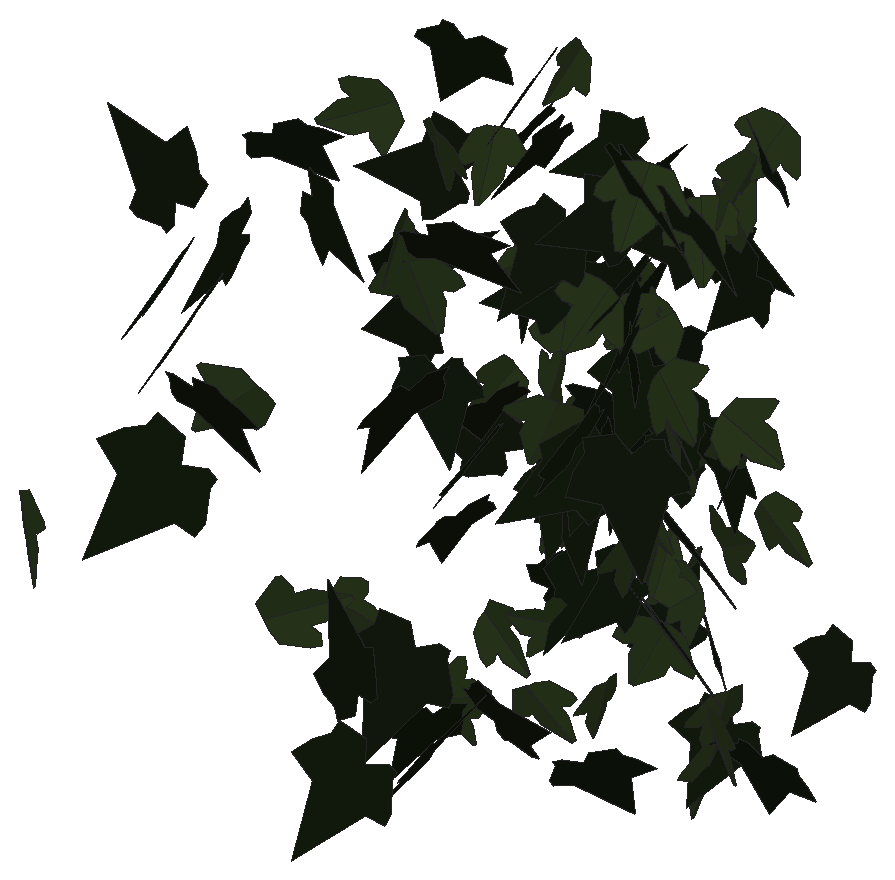
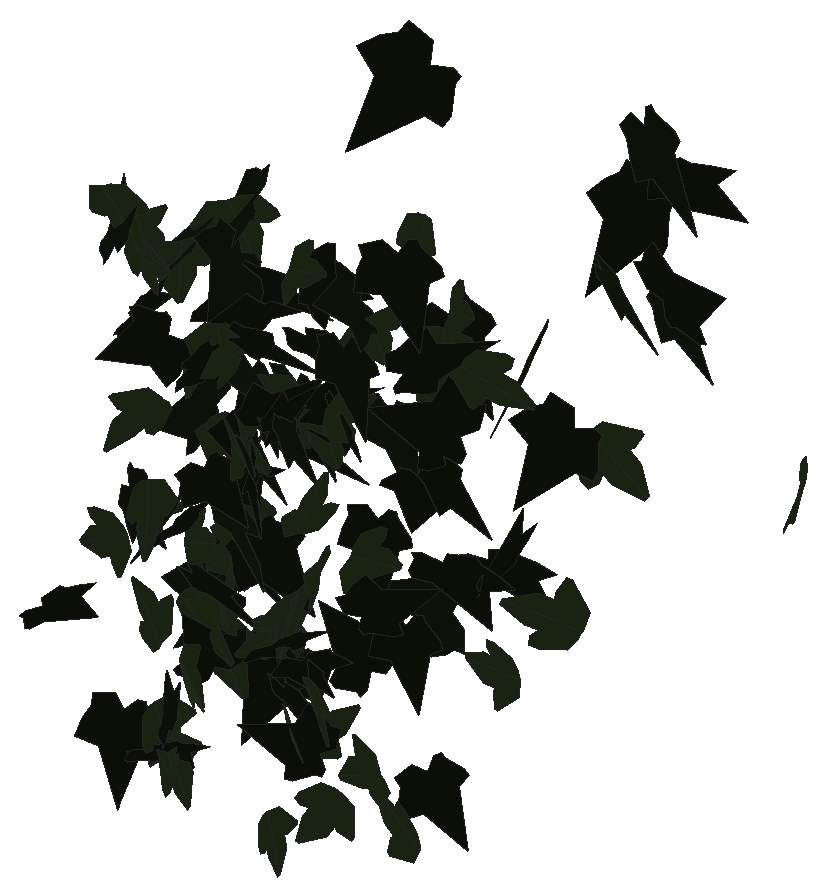
# SketchUp Ruby script. Lengths in inches.
U = 1.inch
M = Sketchup.active_model
def pt(a) = Geom::Point3d.new(a.map { |v| v * U })
def face(e, loops, mat)
  f = e.add_face(loops[0].map { |a| pt(a) })
  loops[1..].each { |l| e.add_face(l.map { |a| pt(a) }).erase! }
  f.material = f.back_material = mat if mat
  f
end
# faces: each face lists its corners as indices into pts; further lists are holes
def faces(e, pts, list, mat = nil) = list.each { |f| face(e, (f[0].is_a?(Array) ? f : [f]).map { |l| l.map { |i| pts[i] } }, mat) }
# xy, xz, yz: faces in a plane at the given z, y or x. An outline is a flat list of corners, or four numbers for a rectangle; further outlines are holes
def ring(l) = l.size == 4 ? [[l[0], l[1]], [l[2], l[1]], [l[2], l[3]], [l[0], l[3]]] : l.each_slice(2).to_a
def flat(e, list, mat, &to3) = list.each { |f| face(e, (f[0].is_a?(Array) ? f : [f]).map { |l| ring(l).map { |u, v| to3.(u, v) } }, mat) }
def xy(e, z, list, mat = nil) = flat(e, list, mat) { |x, y| [x, y, z] }
def xz(e, y, list, mat = nil) = flat(e, list, mat) { |x, z| [x, y, z] }
def yz(e, x, list, mat = nil) = flat(e, list, mat) { |y, z| [x, y, z] }
def lines(e, pts, list) = list.each { |a, b| e.add_line(pt(pts[a]), pt(pts[b])) }
# prism: a flat outline (further loops are holes) pulled along v
def prism(e, loops, v, mat = nil)
  f = face(e, loops, mat); d = Geom::Vector3d.new(v.map { |x| x * U })
  f.pushpull(f.normal.samedirection?(d) ? d.length : -d.length)
end
def box(e, o, s, mat = nil) = prism(e, [[o, [o[0] + s[0], o[1], o[2]], [o[0] + s[0], o[1] + s[1], o[2]], [o[0], o[1] + s[1], o[2]]]], [0, 0, s[2]], mat)
def at(x, y, z, deg = 0) = Geom::Transformation.translation(pt([x, y, z])) * Geom::Transformation.rotation(ORIGIN, Z_AXIS, deg.degrees)
def axes(o, x, y, z) = Geom::Transformation.new([*x, 0, *y, 0, *z, 0, *pt(o).to_a, 1])
def part(name) = M.definitions.add(name)
# library, detail: a bought-in or finely detailed component or shape, given as its bounding box
def library(name, o, s) = part(name).tap { |d| box(d.entities, o, s) }
def detail(e, o, s) = box(e.add_group.entities, o, s)
def put(e, d, t, mat = nil) = e.add_instance(d, t).tap { |i| i.material = mat if mat }
def group(e, t, mat = nil) = e.add_group.tap { |g| g.transformation = t; g.material = mat if mat }.entities
root = M.entities
M.materials.add("efeu1").color = [18, 25, 13]
M.materials.add("efeu2").color = [43, 57, 29]
c1 = part("ivyleaf_9")
p = [[1.54,2.16,1.25],[1.36,2.04,1.19],[-0.21,0.99,0.68],[-0.71,1.11,0.82],[-0.85,0.86,0.67],[-0.8,0.17,0.21],
  [-0.9,-0.01,0.1],[-0.67,-0.16,-0.02],[-0.08,-0.08,-0.05],[-0.03,-0.6,-0.4],[0.65,-0.88,-0.66],[0.83,-0.6,-0.49],
  [1.29,-0.42,-0.43],[1.8125,-0.07,-0.26],[1.21,0.44,0.15]]
faces(c1.entities,p,[[0,1,2,3,4,5,6,7,8,9,10,11,12,13,14]],"efeu1")
c2 = part("ivyleaf_10")
p = [[0,0.5,-0.03],[-0.0625,2.02,-0.43],[-0.19,2.01,-0.46],[-0.54,1.05,-0.29],[-0.52,0.625,-0.18],[-0.83,0.76,-0.28],
  [-1.16,0.64,-0.33],[-1.15,0.33,-0.24],[-0.77,-0.39,0.02],[-0.3,-0.51,0.16],[0.04,-0.48,0.23],[-0.02,2.01,-0.4375],
  [-0.06,2.01,-0.43],[0.04,-0.49,0.23],[0.67,-0.49,0.14],[1.38,0.36,-0.2],[1.375,0.51,-0.24],[0.81,0.65,-0.19],
  [0.62,0.59,-0.15],[0.6,1.09,-0.28],[0.5,1.23,-0.31]]
faces(c2.entities,p,[[0,1,2,3,4,5,6,7,8,9,10],[11,12,0,13,14,15,16,17,18,19,20]],"efeu2")
put(root,c1,axes([502.58,109.68,200.72],[-1.12448,-0.74552,0.3301],[-0.2858,-0.17561,-1.33175],[0.82712,-1.07423,-0.01139]))
put(root,c1,axes([501.1,112.36,204.29],[-0.7784,0.97057,-0.39309],[0.24336,-0.30345,-1.25727],[-1.09825,-0.75515,0.00001]))
put(root,c1,axes([501.125,112.48,201.625],[1.28442,0.17447,-0.3013],[-0.30972,-0.0411,-1.25008],[-0.19359,1.22336,0.00097]))
put(root,c2,axes([493.45,113.83,194.24],[-0.39891,0.91131,-0.49784],[0.20278,-0.4404,-1.02262],[-1.09308,-0.41427,-0.00803]))
put(root,c1,axes([504.72,115.95,188.35],[-1.14523,-0.49988,-0.02559],[0.0231,0.01234,-1.2192],[0.54003,-1.06061,-0.00212]))
put(root,c1,axes([496.22,117.38,201.86],[-0.6941,0.75659,-0.35945],[0.22061,-0.27983,-1.03212],[-0.87083,-0.67394,0.02503]))
put(root,c1,axes([506.59,117.12,206.83],[1.24321,0.52526,0.11586],[0.07008,0.12552,-1.3128],[-0.57565,1.14967,0.09039]))
put(root,c1,axes([502.87,117.99,189.51],[-0.31457,-0.86412,0.68269],[0.21886,0.6244,0.94834],[-1.15137,0.35478,-0.00626]))
put(root,c1,axes([497.61,118.89,202.94],[-0.9682,0.4916,-0.3634],[0.31268,-0.19839,-1.06277],[-0.57143,-0.9415,0.03419]))
put(root,c1,axes([504.9,118.04,187.32],[-0.23729,1.03065,-0.31438],[-0.06927,0.29541,1.09596],[1.15792,0.22888,0.00114]))
put(root,c1,axes([503.63,119.76,190.27],[-1.1445,-0.59034,-0.29556],[0.2678,0.13885,-1.26158],[0.65497,-1.08834,-0.00063]))
put(root,c1,axes([503.72,119.43,199.4],[-0.28753,0.99191,-0.63209],[0.14608,-0.59287,-1.0679],[-1.24785,-0.29796,0.02063]))
put(root,c2,axes([497.17,119.74,197],[-0.65814,-0.39458,0.80063],[-0.66489,-0.46373,-0.75402],[0.65635,-0.86542,0.03899]))
put(root,c1,axes([494.78,119.24,203.17],[-0.07387,0.16981,1.26175],[-0.9393,0.84901,-0.17458],[-0.93176,-0.86935,0.07597]))
put(root,c2,axes([498.64,119.69,189.78],[-0.30008,-0.31215,0.99531],[0.67558,0.72433,0.43458],[-0.8518,0.68444,-0.00597]))
put(root,c1,axes([510.7,121.53,198.65],[-0.42664,-1.05008,-0.53356],[0.14703,0.49652,-1.16594],[1.25361,-0.41561,-0.04484]))
put(root,c1,axes([504.47,121.55,196.39],[-0.46469,1.05397,0.07174],[-0.02966,0.06329,-1.18395],[-1.14033,-0.43114,0.00156]))
put(root,c1,axes([504.78,122.39,187.17],[0.11824,-0.4021,0.99356],[0.82864,-0.61447,-0.36042],[0.75267,0.73966,0.24072]))
put(root,c2,axes([498.83,122.57,189.05],[-0.10427,0.04499,-0.96535],[0.9176,-0.3738,-0.11075],[-0.40661,-0.8551,-0.00238]))
put(root,c2,axes([500.64,123.125,202.36],[-0.12804,0.53057,-0.80239],[-0.0198,-0.77885,-0.5541],[-1.01107,-0.05194,0.11246]))
put(root,c1,axes([508.03,122.69,186.64],[0.8456,0.75683,-0.05717],[-0.04278,-0.03812,-1.13251],[-0.81841,0.78396,0.00013]))
put(root,c2,axes([500.99,123.17,200.95],[-1.0217,-0.4777,-0.27537],[0.26785,0.0961,-1.10186],[0.52554,-0.97766,0.02624]))
put(root,c1,axes([507.25,123.02,197.17],[-0.57036,1.00267,0.20462],[-0.15002,0.14897,-1.1773],[-1.09329,-0.54352,0.05479]))
put(root,c1,axes([497.16,123.13,202.18],[0.78046,-0.5228,-0.7206],[-0.58139,0.4373,-0.92706],[0.73537,0.90059,0.03185]))
put(root,c1,axes([510.3125,123.64,195.68],[0.93816,-0.72233,0.31366],[0.26081,-0.18126,-1.17485],[0.80415,0.90149,0.0151]))
put(root,c1,axes([506.99,124.13,196.03],[-1.19107,-0.1307,0.24865],[-0.24665,-0.10024,-1.15262],[0.1605,-1.124,0.07388]))
put(root,c1,axes([500.93,124.04,185.1875],[-0.10999,0.70293,-0.64495],[0.05457,-0.61877,-0.73806],[-1.0109,-0.10988,0.03033]))
put(root,c2,axes([505.6,124.12,197.34],[-0.72728,-0.6263,0.36516],[-0.26936,-0.24736,-0.95636],[0.72716,-0.71803,0.01096]))
put(root,c2,axes([501.51,123.8,205.4375],[-0.89854,0.37381,0.22973],[-0.2145,0.09692,-0.94856],[-0.417,-0.85533,-0.00709]))
put(root,c1,axes([507.2,125.03,196.22],[0.24883,-0.17622,-1.1552],[1.0631,-0.51682,0.29761],[-0.5875,-1.00984,0.04927]))
put(root,c1,axes([500.62,124.75,196.65],[-0.52574,-0.57982,-0.59905],[0.4189,0.42623,-0.78712],[0.77694,-0.62216,0.01903]))
put(root,c1,axes([508.86,125.45,190.45],[0.69979,-0.69154,0.50361],[0.36067,-0.35067,-0.98556],[0.83739,0.72894,0.00364]))
put(root,c2,axes([507.82,125.28,193.22],[0.00137,-1.07638,-0.0221],[0.02048,0.02126,-1.11926],[1.16254,0.00089,0.01975]))
put(root,c1,axes([507.43,125.55,191.58],[-1.10582,0.27068,-0.05513],[0.05405,-0.01809,-1.10144],[-0.29294,-1.02512,0.00488]))
put(root,c2,axes([509.33,124.99,199.16],[0.05607,0.98769,0.41875],[-0.02751,0.40415,-1.02763],[-1.15161,0.03843,0.04493]))
put(root,c1,axes([499.38,125.53,197.84],[-0.03734,-0.03674,-1.00301],[-0.98172,-0.32307,0.04669],[-0.35028,0.90937,-0.02393]))
put(root,c1,axes([500.73,125.49,191.39],[-0.02288,0.90141,-0.22399],[0.00734,-0.21527,-0.93772],[-1.0009,-0.02219,-0.00176]))
put(root,c1,axes([498.8125,125.25,199.3],[0.23621,0.03081,1.07714],[1.0338,0.39927,-0.22258],[-0.42845,0.98037,0.05679]))
put(root,c2,axes([507.46,126.11,205.13],[0.94861,0.58598,-0.30189],[-0.24738,-0.1796,-1.09787],[-0.66151,0.90746,-0.02234]))
put(root,c1,axes([506.79,126.09,205.58],[0.89346,-0.73775,0.00578],[0.01274,0.00487,-1.15272],[0.79669,0.82728,0.01194]))
put(root,c1,axes([507.59,126.01,190.54],[1.02866,-0.41694,-0.07841],[-0.07453,0.03036,-1.08131],[0.45149,0.95496,0.00015]))
put(root,c1,axes([503.85,126.64,201.77],[-1.11197,-0.28718,-0.12745],[0.13375,0.01205,-1.11144],[0.30955,-1.0368,0.02238]))
put(root,c2,axes([499.76,126.59,184.35],[0.42031,-0.22573,-0.95174],[0.83402,-0.49132,0.46758],[-0.58367,-0.8646,-0.01723]))
put(root,c1,axes([499.46,127,202.22],[-0.3706,-0.18815,1.0336],[-0.92774,-0.4999,-0.40689],[0.57678,-0.92498,0.00965]))
put(root,c1,axes([506.21,126.65,203.17],[-0.90525,0.00119,0.44716],[-0.46433,0.00772,-0.8717],[-0.00495,-0.942,-0.00658]))
put(root,c1,axes([503.42,127,199.45],[-0.40564,-0.24244,0.7561],[-0.59663,-0.4755,-0.46173],[0.57367,-0.66597,0.05442]))
put(root,c1,axes([501.48,126.05,195.39],[0.06004,0.90499,-0.13327],[-0.01397,-0.12759,-0.94295],[-0.98704,0.05685,0.00524]))
put(root,c1,axes([493.28,126.11,201.74],[0.9241,0.6454,0.07882],[0.0624,0.04926,-1.11462],[-0.69905,0.85758,0.0047]))
put(root,c2,axes([507.67,126.62,189.1875],[0.96908,0.27132,-0.42611],[-0.5057,0.21322,-0.91964],[-0.16106,0.9631,0.32364]))
put(root,c1,axes([503.08,127.36,204.74],[-0.47729,0.08759,-0.84618],[0.4477,-0.77332,-0.32075],[-0.76202,-0.5092,0.34156]))
put(root,c2,axes([506.6875,127.47,191.3],[-0.04603,0.0681,1.02388],[0.71803,-0.72624,0.08218],[0.78763,0.66605,-0.01508]))
put(root,c1,axes([508.3,127.09,204.24],[0.64463,-0.86424,0.08166],[0.1436,-0.0031,-1.08662],[0.92616,0.60202,0.11164]))
put(root,c2,axes([504.94,127.09,199.71],[1.05144,-0.1384,-0.43847],[-0.45035,0.06228,-1.02268],[0.16388,1.0591,0.00284]))
put(root,c2,axes([501.9,127.67,199.87],[-0.04984,0.09869,0.91187],[0.11942,-0.87043,0.10794],[0.94541,0.11515,0.03443]))
put(root,c2,axes([502.82,127.58,187.53],[-0.25361,-0.23566,-0.78206],[-0.49996,-0.59375,0.34386],[-0.68876,0.51777,0.03836]))
put(root,c2,axes([496.35,127.23,203.36],[0.51511,0.07657,-0.91858],[-0.94935,-0.08957,-0.50174],[-0.1245,0.99979,0.0254]))
put(root,c2,axes([500.76,127.22,203.64],[0.4952,0.74483,-0.28588],[-0.15293,-0.23562,-0.90963],[-0.8437,0.47988,-0.00291]))
put(root,c2,axes([506.36,127.18,193.24],[-0.6763,0.21591,-0.64796],[0.62528,-0.23118,-0.6885],[-0.34083,-0.85256,0.0226]))
put(root,c2,axes([500.62,127.33,186.83],[0.44528,-0.00951,0.87079],[0.90431,-0.00285,-0.42884],[0.0073,0.9333,0.00756]))
put(root,c1,axes([500.75,127.6,192.86],[-0.14393,0.01037,0.93443],[-0.96667,-0.0815,-0.13709],[0.08544,-0.90466,0.02306]))
put(root,c1,axes([501.87,127.57,200.02],[-0.58164,0.00955,-0.733],[0.76027,-0.03802,-0.55996],[-0.03888,-0.8862,0.01612]))
put(root,c2,axes([500.78,127.88,195.17],[0.25414,0.47109,-0.85162],[-0.3826,-0.7383,-0.5476],[-0.94583,0.42523,-0.00732]))
put(root,c2,axes([502.4,127.31,185.03],[-0.7905,-0.13669,-0.46765],[0.47646,0.0871,-0.77437],[0.17499,-0.8546,-0.00413]))
put(root,c1,axes([499.56,127.38,206.64],[0.55084,0.50592,-0.78942],[-0.60352,-0.51409,-0.74686],[-0.7787,0.75632,0.02041]))
put(root,c2,axes([508.63,127.49,203.76],[0.70784,0.82332,-0.01056],[-0.01263,-0.00367,-1.09441],[-0.88917,0.65547,0.00714]))
put(root,c2,axes([508.63,127.85,184.85],[0.11469,-0.93658,0.25158],[0.08579,-0.23409,-0.97885],[1.04117,0.12246,0.05294]))
put(root,c2,axes([507,127.5,190.43],[0.9435,-0.11444,-0.11594],[0.12203,0.00448,0.91611],[-0.12199,-0.88069,0.01973]))
put(root,c2,axes([508.07,127.48,190.52],[0.65622,-0.32087,-0.84184],[-0.78722,0.35252,-0.71435],[0.51443,0.94876,-0.01929]))
put(root,c2,axes([510.1875,127.16,197.1875],[0.29179,0.65255,0.71509],[0.30225,0.62819,-0.73439],[-0.97814,0.38878,-0.01361]))
put(root,c1,axes([507.28,127.38,188.62],[-0.44382,-0.27337,0.779],[0.73365,0.32123,0.50952],[-0.45094,0.79168,0.06225]))
put(root,c1,axes([505.71,127.3,200.16],[-0.38947,0.94421,0.24992],[-0.13603,0.20891,-1.05025],[-1.04342,-0.37967,0.04364]))
put(root,c1,axes([506.48,127.08,204.21],[0.24123,0.85975,0.54896],[0.05482,0.53037,-0.92075],[-1.08819,0.21731,0.07531]))
put(root,c1,axes([509.69,128.66,201.48],[-0.23966,-0.66441,0.66658],[-0.21531,-0.60915,-0.7285],[0.9735,-0.29829,0.00297]))
put(root,c2,axes([508.75,127.86,186.16],[-0.79278,0.59434,-0.27053],[0.24236,-0.13594,-0.98163],[-0.65742,-0.76683,-0.03565]))
put(root,c1,axes([505.38,128.16,198.3],[-0.80542,0.45611,-0.57249],[0.48894,-0.31432,-0.90871],[-0.59753,-0.872,0.02811]))
put(root,c1,axes([503.54,128.21,189.27],[-0.95919,-0.01677,-0.34022],[0.35243,0.03683,-0.92334],[0.03073,-0.94575,-0.02992]))
put(root,c1,axes([510.875,127.68,185.61],[0.76673,0.43011,-0.64531],[-0.63535,-0.21869,-0.85767],[-0.51106,0.91716,0.09812]))
put(root,c1,axes([504.38,128.41,199.17],[0.12332,0.00384,0.84979],[-0.84613,-0.23386,0.115],[0.25069,-0.79121,-0.02987]))
put(root,c1,axes([513.29,128.75,189.32],[-0.51707,-0.7657,0.35319],[-0.19734,-0.29292,-0.92393],[0.81981,-0.55344,0.00036]))
put(root,c1,axes([508.69,128.78,185.5],[-0.69008,-0.71813,0.07708],[0.11175,-0.18906,-0.97728],[0.77165,-0.61484,0.21047]))
put(root,c2,axes([508.75,128.37,186.55],[-0.09371,-0.96899,0.11336],[0.00371,-0.10973,-1.01169],[1.05311,-0.08583,0.01365]))
put(root,c1,axes([505.62,128.78,196.77],[-0.54789,-0.88155,0.05387],[0.02227,-0.07155,-1.05632],[0.95345,-0.5049,0.05563]))
put(root,c1,axes([501.1,127.52,204.55],[-0.44424,0.73222,-0.53251],[-0.31225,0.42428,0.87255],[0.91305,0.50135,0.03931]))
put(root,c2,axes([509.14,129.02,204.84],[0.01445,-0.68719,0.67884],[0.15429,-0.64388,-0.70803],[1.01191,0.10799,0.09826]))
put(root,c2,axes([509.66,128.18,203.48],[0.38958,0.05518,0.93127],[-0.943,0.24336,0.35021],[-0.22264,-0.9342,0.14624]))
put(root,c1,axes([505.34,128.16,197.73],[0.18331,-0.01166,-1.06851],[-1.10022,0.13373,-0.17661],[0.14454,1.03271,0.01081]))
put(root,c2,axes([502.55,128.87,187.58],[0.37519,-0.43577,-0.58978],[0.4143,-0.41855,0.57889],[-0.65189,-0.51681,0.02847]))
put(root,c2,axes([505.83,128.91,198.5625],[0.68721,0.03595,-0.76081],[-0.78722,-0.06391,-0.66263],[-0.07754,0.96745,-0.01551]))
put(root,c1,axes([504.25,128.71,194.92],[0.06501,0.46827,-0.92524],[-0.81571,-0.56717,-0.36362],[-0.71664,0.68806,0.32996]))
put(root,c1,axes([502.41,129.16,191.34],[-0.56614,-0.38702,-0.71723],[0.74413,0.18258,-0.65124],[0.41919,-0.84679,0.18739]))
put(root,c2,axes([502.29,129.36,206.15],[0.05947,0.46358,-0.76259],[-0.21328,-0.70875,-0.48143],[-0.91232,0.19591,0.06284]))
put(root,c2,axes([510.09,129.08,193.23],[-0.53152,0.11996,-0.80488],[0.7486,-0.35875,-0.51624],[-0.39371,-0.84407,0.10502]))
put(root,c1,axes([505.18,128.16,198.28],[0.08377,0.07173,1.0772],[0.38749,0.97281,-0.09801],[-1.05222,0.36396,0.04967]))
put(root,c1,axes([501.9375,129.35,191.46],[-0.49254,-0.7185,-0.13419],[0.07819,0.10687,-0.88505],[0.78451,-0.46175,0.00396]))
put(root,c1,axes([507.98,129.56,194.3],[0.19612,-0.85419,0.446],[0.11204,-0.41633,-0.9081],[1.02616,0.20871,0.01391]))
put(root,c1,axes([505.53,128.61,195.7],[-0.4932,0.89358,0.19853],[-0.10903,0.16276,-1.04352],[-0.9808,-0.46743,0.01617]))
put(root,c1,axes([500.71,128.72,203.3],[-0.26828,0.96495,-0.09518],[0.02598,-0.08831,-1.03626],[-1.0465,-0.24956,-0.00132]))
put(root,c1,axes([506.4,129.73,201.11],[0.04917,-0.63839,-0.56197],[0.14899,-0.52801,0.66085],[-0.89091,-0.12353,0.0795]))
put(root,c2,axes([503.42,129.21,184.71],[0.01543,-0.82419,0.0109],[0.01005,-0.01032,-0.85723],[0.89014,0.0144,0.00949]))
put(root,c2,axes([507.09,128.71,193.87],[-0.29121,0.30935,-0.89794],[-0.6662,0.60481,0.42571],[0.73301,0.67259,0.03018]))
put(root,c1,axes([501.78,128.89,187.9],[0.33391,-0.02752,0.84932],[0.88247,0.01518,-0.32119],[-0.00482,0.87309,0.03235]))
put(root,c1,axes([509.51,129.8,204.8125],[-0.19218,-0.26955,0.90986],[0.20184,-0.88317,-0.24346],[0.96786,0.13066,0.23143]))
put(root,c1,axes([507.33,129.73,187.3],[0.03438,-0.22607,0.82223],[0.17469,-0.77402,-0.23696],[0.87072,0.16421,0.01508]))
put(root,c1,axes([506.98,129.85,195.06],[-0.23197,-0.72392,0.33843],[-0.06564,-0.32113,-0.78468],[0.85468,-0.22115,0.03159]))
put(root,c2,axes([501.96,129.28,196.66],[0.1673,0.89511,0.20574],[-0.04574,-0.19343,0.94471],[0.98899,-0.16036,0.00889]))
put(root,c2,axes([501.67,129.31,190.47],[0.75639,-0.56315,-0.22747],[-0.18426,0.13685,-0.93464],[0.6259,0.72084,-0.00026]))
put(root,c1,axes([502.82,129.92,200.18],[-0.11637,-0.1608,0.79739],[-0.45147,-0.64274,-0.20129],[0.71555,-0.43168,0.00268]))
put(root,c2,axes([503.01,129.01,192.02],[-0.36649,-0.25143,-0.75419],[0.69965,0.33139,-0.43477],[0.44454,-0.72885,0.06249]))
put(root,c2,axes([509.92,129.45,206.1875],[0.96424,-0.0799,-0.42586],[-0.43789,0.0617,-0.93193],[0.10616,0.9803,0.02395]))
put(root,c1,axes([502.6,129.61,200.35],[-0.67761,0.47334,-0.49463],[0.41303,-0.28277,-0.81737],[-0.59547,-0.73478,-0.00408]))
put(root,c1,axes([508.88,129.75,195.67],[-0.55827,0.42688,-0.71591],[0.56552,-0.44693,-0.69716],[-0.66742,-0.73575,0.00812]))
put(root,c2,axes([504.36,129.875,198.7],[-0.03607,-0.05533,-0.89747],[0.62315,-0.64466,0.01976],[-0.6956,-0.57465,0.06424]))
put(root,c2,axes([508.41,129.39,195.41],[-0.17113,-0.95037,-0.26109],[0.06224,0.24487,-1.00189],[1.05978,-0.16784,0.01668]))
put(root,c2,axes([502.4,129.17,193.09],[-0.04016,0.72915,0.33901],[-0.04398,0.32417,-0.75895],[-0.86147,-0.05054,0.02294]))
put(root,c1,axes([502.51,130.17,192.23],[-0.46242,-0.85176,0.14462],[0.10116,-0.20018,-0.97522],[0.92657,-0.40323,0.17865]))
put(root,c2,axes([506.375,129.91,189.87],[0.45712,-0.75489,0.3674],[0.18517,-0.30888,-0.90007],[0.88089,0.45666,-0.00146]))
put(root,c1,axes([506.03,129.84,193.46],[-1.0548,0.03273,0.07202],[-0.07553,-0.01973,-1.01604],[-0.03374,-0.97892,0.02289]))
put(root,c2,axes([501.62,128.92,194.7],[0.01646,0.34987,-0.82733],[-0.08474,0.79294,0.36112],[0.93474,0.06573,0.0473]))
put(root,c2,axes([505.3125,128.96,201.6],[0.0801,-0.04759,0.83816],[-0.22946,0.77964,0.06821],[-0.84118,-0.2172,0.0612]))
put(root,c2,axes([507.67,129.88,190.86],[-0.58236,0.08663,0.82012],[0.83518,-0.15538,0.56769],[0.1912,0.94259,0.0182]))
put(root,c1,axes([505.61,129.87,197.6],[0.08258,0.39993,-0.69517],[-0.17675,-0.64841,-0.42294],[-0.82248,0.17949,0.02109]))
put(root,c2,axes([502.17,129.62,193.77],[-0.00149,0.98623,-0.02181],[0.00449,-0.02097,-1.02567],[-1.06536,-0.00147,-0.00429]))
put(root,c1,axes([503.96,129.98,203.18],[-0.83446,0.05527,0.44593],[-0.46551,-0.03045,-0.80369],[-0.03617,-0.88313,0.05562]))
put(root,c1,axes([507.63,129.51,201.79],[0.01102,0.03156,-0.96983],[0.72502,0.64746,0.03043],[0.69988,-0.67121,-0.01625]))
put(root,c2,axes([502.22,129.71,193.55],[0.19764,0.96504,0.00572],[0.003,0.00507,-1.02153],[-1.04226,0.18301,-0.00185]))
